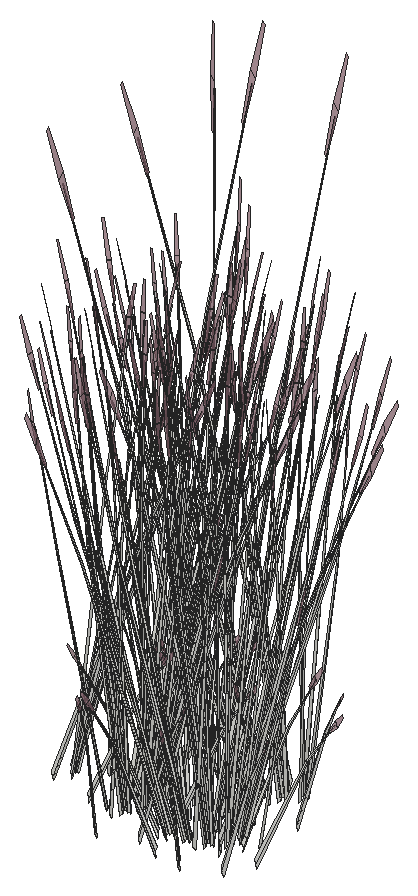
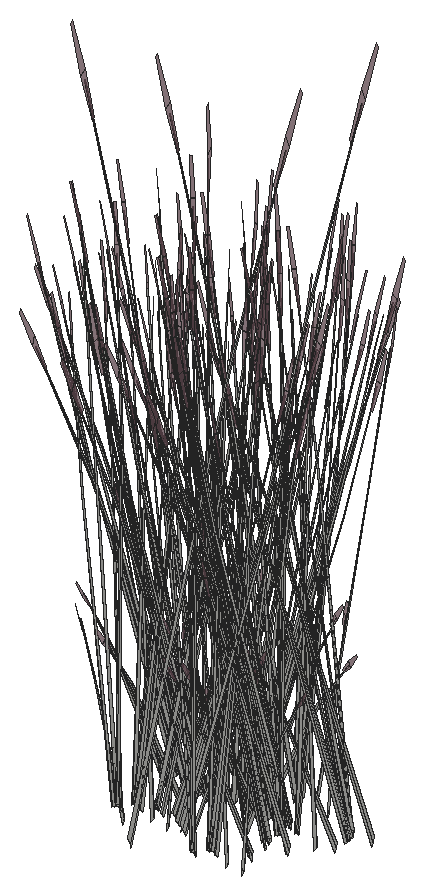
# SketchUp Ruby script. Lengths in inches.
U = 1.inch
M = Sketchup.active_model
def pt(a) = Geom::Point3d.new(a.map { |v| v * U })
def face(e, loops, mat)
  f = e.add_face(loops[0].map { |a| pt(a) })
  loops[1..].each { |l| e.add_face(l.map { |a| pt(a) }).erase! }
  f.material = f.back_material = mat if mat
  f
end
# faces: each face lists its corners as indices into pts; further lists are holes
def faces(e, pts, list, mat = nil) = list.each { |f| face(e, (f[0].is_a?(Array) ? f : [f]).map { |l| l.map { |i| pts[i] } }, mat) }
# xy, xz, yz: faces in a plane at the given z, y or x. An outline is a flat list of corners, or four numbers for a rectangle; further outlines are holes
def ring(l) = l.size == 4 ? [[l[0], l[1]], [l[2], l[1]], [l[2], l[3]], [l[0], l[3]]] : l.each_slice(2).to_a
def flat(e, list, mat, &to3) = list.each { |f| face(e, (f[0].is_a?(Array) ? f : [f]).map { |l| ring(l).map { |u, v| to3.(u, v) } }, mat) }
def xy(e, z, list, mat = nil) = flat(e, list, mat) { |x, y| [x, y, z] }
def xz(e, y, list, mat = nil) = flat(e, list, mat) { |x, z| [x, y, z] }
def yz(e, x, list, mat = nil) = flat(e, list, mat) { |y, z| [x, y, z] }
def lines(e, pts, list) = list.each { |a, b| e.add_line(pt(pts[a]), pt(pts[b])) }
# prism: a flat outline (further loops are holes) pulled along v
def prism(e, loops, v, mat = nil)
  f = face(e, loops, mat); d = Geom::Vector3d.new(v.map { |x| x * U })
  f.pushpull(f.normal.samedirection?(d) ? d.length : -d.length)
end
def box(e, o, s, mat = nil) = prism(e, [[o, [o[0] + s[0], o[1], o[2]], [o[0] + s[0], o[1] + s[1], o[2]], [o[0], o[1] + s[1], o[2]]]], [0, 0, s[2]], mat)
def at(x, y, z, deg = 0) = Geom::Transformation.translation(pt([x, y, z])) * Geom::Transformation.rotation(ORIGIN, Z_AXIS, deg.degrees)
def axes(o, x, y, z) = Geom::Transformation.new([*x, 0, *y, 0, *z, 0, *pt(o).to_a, 1])
def part(name) = M.definitions.add(name)
# library, detail: a bought-in or finely detailed component or shape, given as its bounding box
def library(name, o, s) = part(name).tap { |d| box(d.entities, o, s) }
def detail(e, o, s) = box(e.add_group.entities, o, s)
def put(e, d, t, mat = nil) = e.add_instance(d, t).tap { |i| i.material = mat if mat }
def group(e, t, mat = nil) = e.add_group.tap { |g| g.transformation = t; g.material = mat if mat }.entities
root = M.entities
M.materials.add("LightPink_Translucent").color = [144, 107, 117]
M.materials["LightPink_Translucent"].alpha = 0.75
c1 = part("blade")
p = [[2.15,0.21,22],[0,0.17,0],[0.09,0.45,0],[2.18,0.31,22],[2.29,0.31,22],[0.38,0.45,0],
  [2.48,0.24,33],[2.49,0.24,33],[2.48,0.22,33]]
faces(c1.entities,p,[[0,1,2,3],[4,5,2,3],[6,3,4,7],[8,0,3,6]])
c2 = part("seeds")
p = [[0.3,-0.1,1.38],[-0.01,-0.03,1.59],[-0.01,-0.03,0.03],[0.14,-0.07,-0.07],[0.29,-0.03,3],[0.15,0.01,3.11]]
faces(c2.entities,p,[[0,1,2,3],[1,0,4,5]],"LightPink_Translucent")
c3 = part("blade with seeds")
put(c3.entities,c1,at(0,0,0))
put(c3.entities,c2,axes([2.4,0.25,30.99],[1.5799,-0.05474,1.17369],[-0.12525,1.92788,0.29478],[-0.07173,-0.02425,1.56792]))
put(root,c3,axes([338.69,15.14,51.43],[0.11542,0.12546,1.51428],[-0.53333,0.10562,0.12244],[-0.12054,-0.19696,0.64734]))
put(root,c3,axes([340.11,15.23,52.4],[-0.24099,-0.31773,-0.62776],[0.49607,-0.17707,0.07576],[-0.05635,-0.15352,0.88802]))
put(root,c3,axes([335.52,15.54,52.4],[0.01314,-0.36145,-0.62776],[0.55324,0.02428,0.07576],[0.05838,-0.15313,0.88802]))
put(root,c3,axes([341.12,15.54,52.4],[0.01314,-0.36145,-0.62776],[0.55324,0.02428,0.07576],[0.05838,-0.15313,0.88802]))
put(root,c3,axes([334.5625,14.96,52],[0.15222,-0.30049,-0.31292],[0.44409,0.08764,0.40398],[-0.04072,-0.12098,0.77298]))
put(root,c3,axes([340.16,14.96,52],[0.15222,-0.30049,-0.31292],[0.44409,0.08764,0.40398],[-0.04072,-0.12098,0.77298]))
put(root,c3,axes([334.9,15.36,51.43],[-0.09401,0.13431,1.51428],[-0.3944,-0.27795,0.12244],[0.17792,-0.17323,0.64734]))
put(root,c3,axes([340.5,15.36,51.43],[-0.09401,0.13431,1.51428],[-0.3944,-0.27795,0.12244],[0.17792,-0.17323,0.64734]))
put(root,c3,axes([339.93,15.17,52.14],[-0.49634,-0.09796,-0.45151],[0.17013,-0.33585,-0.34973],[-0.04551,-0.13522,0.86392]))
put(root,c3,axes([334.64,14.33,50.44],[0.06477,0.22786,1.01491],[-0.35932,-0.1262,0.74569],[0.03867,-0.11667,0.22354]))
put(root,c3,axes([340.24,14.33,50.44],[0.06477,0.22786,1.01491],[-0.35932,-0.1262,0.74569],[0.03867,-0.11667,0.22354]))
put(root,c3,axes([335.41,15.42,52.14],[-0.36145,-0.26255,-0.45151],[0.38183,-0.22994,-0.34973],[0.055,-0.1334,0.86392]))
put(root,c3,axes([341.01,15.42,52.14],[-0.36145,-0.26255,-0.45151],[0.38183,-0.22994,-0.34973],[0.055,-0.1334,0.86392]))
put(root,c3,axes([340.36,15.15,52.45],[-0.49409,0.18193,-0.10745],[-0.24281,-0.32289,-0.59638],[-0.06519,-0.13607,0.90619]))
put(root,c3,axes([335.79,15.56,52.45],[-0.55492,-0.01936,-0.10745],[0.01517,-0.36657,-0.59638],[0.03855,-0.14118,0.90619]))
put(root,c3,axes([341.38,15.56,52.45],[-0.55492,-0.01936,-0.10745],[0.01517,-0.36657,-0.59638],[0.03855,-0.14118,0.90619]))
put(root,c3,axes([335.75,15.32,52],[0.34164,-0.20573,-0.31292],[0.3234,0.23491,0.40398],[0.04921,-0.11936,0.77298]))
put(root,c3,axes([341.35,15.32,52],[0.34164,-0.20573,-0.31292],[0.3234,0.23491,0.40398],[0.04921,-0.11936,0.77298]))
put(root,c3,axes([338.39,14.6,50.44],[0.26338,0.136,1.01491],[-0.38358,0.08175,0.74569],[-0.08207,-0.10452,0.22354]))
put(root,c3,axes([339.03,15.32,52.4],[-0.43054,-0.18887,-0.62776],[0.30598,-0.33097,0.07576],[-0.15599,-0.11277,0.88802]))
put(root,c3,axes([338.88,15.07,52],[-0.07798,-0.31474,-0.31292],[0.44579,-0.08311,0.40398],[-0.11974,-0.09019,0.77298]))
put(root,c3,axes([338.83,15.33,52.14],[-0.49824,0.09289,-0.45151],[-0.08716,-0.35177,-0.34973],[-0.13382,-0.10081,0.86392]))
put(root,c3,axes([336.17,16.17,52.4],[0.26374,-0.30832,-0.62776],[0.46217,0.21911,0.07576],[0.15748,-0.11171,0.88802]))
put(root,c3,axes([341.77,16.17,52.4],[0.26374,-0.30832,-0.62776],[0.46217,0.21911,0.07576],[0.15748,-0.11171,0.88802]))
put(root,c3,axes([336.16,16.03,52.14],[-0.12971,-0.3568,-0.45151],[0.49122,-0.06241,-0.34973],[0.14077,-0.09583,0.86392]))
put(root,c3,axes([341.76,16.03,52.14],[-0.12971,-0.3568,-0.45151],[0.49122,-0.06241,-0.34973],[0.14077,-0.09583,0.86392]))
put(root,c3,axes([336.39,16.28,52.45],[-0.46706,-0.21546,-0.10745],[0.26908,-0.31203,-0.59638],[0.13196,-0.10846,0.90619]))
put(root,c3,axes([341.99,16.28,52.45],[-0.46706,-0.21546,-0.10745],[0.26908,-0.31203,-0.59638],[0.13196,-0.10846,0.90619]))
put(root,c3,axes([340.06,17.46,50.9375],[0.43633,0.15757,1.33654],[-0.42745,0.33945,0.52853],[-0.19146,-0.20119,1.12046]))
put(root,c3,axes([336.76,15.32,50.44],[-0.16818,0.19891,1.01491],[-0.14456,-0.26725,0.74569],[0.1389,-0.06697,0.22354]))
put(root,c3,axes([342.36,15.32,50.44],[-0.16818,0.19891,1.01491],[-0.14456,-0.26725,0.74569],[0.1389,-0.06697,0.22354]))
put(root,c3,axes([336.52,16.0625,52],[0.43951,-0.05584,-0.31292],[0.11606,0.31924,0.40398],[0.12595,-0.08575,0.77298]))
put(root,c3,axes([342.12,16.0625,52],[0.43951,-0.05584,-0.31292],[0.11606,0.31924,0.40398],[0.12595,-0.08575,0.77298]))
put(root,c3,axes([337.85,15.625,52],[-0.28729,-0.24465,-0.31292],[0.32804,-0.23159,0.40398],[-0.16667,-0.03524,0.77298]))
put(root,c3,axes([337.98,15.87,52.14],[-0.36663,0.25884,-0.45151],[-0.32109,-0.27343,-0.34973],[-0.18628,-0.03938,0.86392]))
put(root,c3,axes([337.16,16.21,50.44],[0.32236,-0.02796,1.01491],[-0.20448,0.24636,0.74569],[-0.1593,-0.03696,0.22354]))
put(root,c3,axes([332.66,18.94,52.4],[0.01314,-0.36145,-0.62776],[0.55324,0.02428,0.07576],[0.05838,-0.15313,0.88802]))
put(root,c3,axes([338.18,15.6,52.45],[-0.02704,0.39739,-0.10745],[-0.51189,-0.01086,-0.59638],[-0.19715,-0.0276,0.90619]))
put(root,c3,axes([330.75,17.12,52.45],[-0.25405,-0.35383,-0.10745],[0.45089,-0.17388,-0.59638],[0.19001,-0.04668,0.90619]))
put(root,c3,axes([336.41,17.12,52.45],[-0.25405,-0.35383,-0.10745],[0.45089,-0.17388,-0.59638],[0.19001,-0.04668,0.90619]))
put(root,c3,axes([342.01,17.12,52.45],[-0.25405,-0.35383,-0.10745],[0.45089,-0.17388,-0.59638],[0.19001,-0.04668,0.90619]))
put(root,c3,axes([330.73,16.82,52.14],[0.13679,-0.35544,-0.45151],[0.46898,0.12183,-0.34973],[0.18882,-0.03259,0.86392]))
put(root,c3,axes([336.39,16.82,52.14],[0.13679,-0.35544,-0.45151],[0.46898,0.12183,-0.34973],[0.18882,-0.03259,0.86392]))
put(root,c3,axes([341.98,16.82,52.14],[0.13679,-0.35544,-0.45151],[0.46898,0.12183,-0.34973],[0.18882,-0.03259,0.86392]))
put(root,c3,axes([332.04,18.76,51.43],[-0.09401,0.13431,1.51428],[-0.3944,-0.27795,0.12244],[0.17792,-0.17323,0.64734]))
put(root,c3,axes([330.64,16.95,52.4],[0.44368,-0.17257,-0.62776],[0.24726,0.35524,0.07576],[0.21437,-0.04035,0.88802]))
put(root,c3,axes([336.3,16.95,52.4],[0.44368,-0.17257,-0.62776],[0.24726,0.35524,0.07576],[0.21437,-0.04035,0.88802]))
put(root,c3,axes([341.9,16.95,52.4],[0.44368,-0.17257,-0.62776],[0.24726,0.35524,0.07576],[0.21437,-0.04035,0.88802]))
put(root,c3,axes([332.89,18.72,52],[0.34164,-0.20573,-0.31292],[0.3234,0.23491,0.40398],[0.04921,-0.11936,0.77298]))
put(root,c3,axes([331.02,16.98,52],[0.41962,0.10901,-0.31292],[-0.12239,0.31802,0.40398],[0.16894,-0.02916,0.77298]))
put(root,c3,axes([336.68,16.98,52],[0.41962,0.10901,-0.31292],[-0.12239,0.31802,0.40398],[0.16894,-0.02916,0.77298]))
put(root,c3,axes([342.27,16.98,52],[0.41962,0.10901,-0.31292],[-0.12239,0.31802,0.40398],[0.16894,-0.02916,0.77298]))
put(root,c3,axes([329.875,16.59,51.43],[-0.20943,0.00885,1.51428],[0.13893,-0.38357,0.12244],[0.29846,0.02372,0.64734]))
put(root,c3,axes([335.53,16.59,51.43],[-0.20943,0.00885,1.51428],[0.13893,-0.38357,0.12244],[0.29846,0.02372,0.64734]))
put(root,c3,axes([341.13,16.59,51.43],[-0.20943,0.00885,1.51428],[0.13893,-0.38357,0.12244],[0.29846,0.02372,0.64734]))
put(root,c3,axes([333.3125,19.57,52.4],[0.26374,-0.30832,-0.62776],[0.46217,0.21911,0.07576],[0.15748,-0.11171,0.88802]))
put(root,c3,axes([333.3,19.43,52.14],[-0.12971,-0.3568,-0.45151],[0.49122,-0.06241,-0.34973],[0.14077,-0.09583,0.86392]))
put(root,c3,axes([333.53,19.68,52.45],[-0.46706,-0.21546,-0.10745],[0.26908,-0.31203,-0.59638],[0.13196,-0.10846,0.90619]))
put(root,c3,axes([331.91,17.04,50.44],[-0.31197,0.06451,1.01491],[0.14684,-0.26661,0.74569],[0.1655,0.01824,0.22354]))
put(root,c3,axes([337.57,17.04,50.44],[-0.31197,0.06451,1.01491],[0.14684,-0.26661,0.74569],[0.1655,0.01824,0.22354]))
put(root,c3,axes([343.16,17.04,50.44],[-0.31197,0.06451,1.01491],[0.14684,-0.26661,0.74569],[0.1655,0.01824,0.22354]))
put(root,c3,axes([337.63,16.64,52.14],[-0.13679,0.35544,-0.45151],[-0.46898,-0.12183,-0.34973],[-0.18882,0.03259,0.86392]))
put(root,c3,axes([337.61,16.33,52.45],[0.25405,0.35383,-0.10745],[-0.45089,0.17388,-0.59638],[-0.19001,0.04668,0.90619]))
put(root,c3,axes([333.9,18.72,50.44],[-0.16818,0.19891,1.01491],[-0.14456,-0.26725,0.74569],[0.1389,-0.06697,0.22354]))
put(root,c3,axes([337.02,17.87,51.47],[-0.09664,-0.32847,-0.03085],[0.45676,-0.07551,-0.13989],[0.09538,0.02082,0.4614]))
put(root,c3,axes([342.62,17.87,51.47],[-0.09664,-0.32847,-0.03085],[0.45676,-0.07551,-0.13989],[0.09538,0.02082,0.4614]))
put(root,c3,axes([330.18,17.86,52.45],[0.02704,-0.39739,-0.10745],[0.51189,0.01086,-0.59638],[0.19715,0.0276,0.90619]))
put(root,c3,axes([335.84,17.86,52.45],[0.02704,-0.39739,-0.10745],[0.51189,0.01086,-0.59638],[0.19715,0.0276,0.90619]))
put(root,c3,axes([341.4375,17.86,52.45],[0.02704,-0.39739,-0.10745],[0.51189,0.01086,-0.59638],[0.19715,0.0276,0.90619]))
put(root,c3,axes([333.66,19.46,52],[0.43951,-0.05584,-0.31292],[0.11606,0.31924,0.40398],[0.12595,-0.08575,0.77298]))
put(root,c3,axes([338.69,21.41,51.43],[0.11542,0.12546,1.51428],[-0.53333,0.10562,0.12244],[-0.12054,-0.19696,0.64734]))
put(root,c3,axes([340.11,21.5,52.4],[-0.24099,-0.31773,-0.62776],[0.49607,-0.17707,0.07576],[-0.05635,-0.15352,0.88802]))
put(root,c3,axes([330.21,17.67,52.4],[0.50473,0.00941,-0.62776],[-0.0339,0.39618,0.07576],[0.21383,0.04181,0.88802]))
put(root,c3,axes([335.86,17.67,52.4],[0.50473,0.00941,-0.62776],[-0.0339,0.39618,0.07576],[0.21383,0.04181,0.88802]))
put(root,c3,axes([341.46,17.67,52.4],[0.50473,0.00941,-0.62776],[-0.0339,0.39618,0.07576],[0.21383,0.04181,0.88802]))
put(root,c3,axes([341.12,21.8125,52.4],[0.01314,-0.36145,-0.62776],[0.55324,0.02428,0.07576],[0.05838,-0.15313,0.88802]))
put(root,c3,axes([340.16,21.23,52],[0.15222,-0.30049,-0.31292],[0.44409,0.08764,0.40398],[-0.04072,-0.12098,0.77298]))
put(root,c3,axes([340.5,21.63,51.43],[-0.09401,0.13431,1.51428],[-0.3944,-0.27795,0.12244],[0.17792,-0.17323,0.64734]))
put(root,c3,axes([339.93,21.4375,52.14],[-0.49634,-0.09796,-0.45151],[0.17013,-0.33585,-0.34973],[-0.04551,-0.13522,0.86392]))
put(root,c3,axes([340.24,20.6,50.44],[0.06477,0.22786,1.01491],[-0.35932,-0.1262,0.74569],[0.03867,-0.11667,0.22354]))
put(root,c3,axes([341.01,21.69,52.14],[-0.36145,-0.26255,-0.45151],[0.38183,-0.22994,-0.34973],[0.055,-0.1334,0.86392]))
put(root,c3,axes([336.7,18.16,50.44],[0.21042,-0.1771,1.01491],[0.08303,0.28036,0.74569],[-0.15207,0.0502,0.22354]))
put(root,c3,axes([330.51,17.83,52],[0.28729,0.24465,-0.31292],[-0.32804,0.23159,0.40398],[0.16667,0.03524,0.77298]))
put(root,c3,axes([336.17,17.83,52],[0.28729,0.24465,-0.31292],[-0.32804,0.23159,0.40398],[0.16667,0.03524,0.77298]))
put(root,c3,axes([341.77,17.83,52],[0.28729,0.24465,-0.31292],[-0.32804,0.23159,0.40398],[0.16667,0.03524,0.77298]))
put(root,c3,axes([337.49,17.39,52],[-0.43951,0.05584,-0.31292],[-0.11606,-0.31924,0.40398],[-0.12595,0.08575,0.77298]))
put(root,c3,axes([333.55,20.52,52.45],[-0.25405,-0.35383,-0.10745],[0.45089,-0.17388,-0.59638],[0.19001,-0.04668,0.90619]))
put(root,c3,axes([333.53,20.22,52.14],[0.13679,-0.35544,-0.45151],[0.46898,0.12183,-0.34973],[0.18882,-0.03259,0.86392]))
put(root,c3,axes([340.36,21.42,52.45],[-0.49409,0.18193,-0.10745],[-0.24281,-0.32289,-0.59638],[-0.06519,-0.13607,0.90619]))
put(root,c3,axes([341.38,21.83,52.45],[-0.55492,-0.01936,-0.10745],[0.01517,-0.36657,-0.59638],[0.03855,-0.14118,0.90619]))
put(root,c3,axes([341.35,21.6,52],[0.34164,-0.20573,-0.31292],[0.3234,0.23491,0.40398],[0.04921,-0.11936,0.77298]))
put(root,c3,axes([338.39,20.87,50.44],[0.26338,0.136,1.01491],[-0.38358,0.08175,0.74569],[-0.08207,-0.10452,0.22354]))
put(root,c3,axes([339.03,21.59,52.4],[-0.43054,-0.18887,-0.62776],[0.30598,-0.33097,0.07576],[-0.15599,-0.11277,0.88802]))
put(root,c3,axes([338.88,21.34,52],[-0.07798,-0.31474,-0.31292],[0.44579,-0.08311,0.40398],[-0.11974,-0.09019,0.77298]))
put(root,c3,axes([335.14,17.2,51.43],[-0.18755,-0.06732,1.51428],[0.38813,-0.28243,0.12244],[0.24191,0.12741,0.64734]))
put(root,c3,axes([340.73,17.2,51.43],[-0.18755,-0.06732,1.51428],[0.38813,-0.28243,0.12244],[0.24191,0.12741,0.64734]))
put(root,c3,axes([335.17,16.32,51.95],[-0.4363,-0.20303,1.22187],[0.46069,-0.31611,0.5272],[0.14077,0.1905,1.18105]))
put(root,c3,axes([340.77,16.32,51.95],[-0.4363,-0.20303,1.22187],[0.46069,-0.31611,0.5272],[0.14077,0.1905,1.18105]))
put(root,c3,axes([333.4375,20.35,52.4],[0.44368,-0.17257,-0.62776],[0.24726,0.35524,0.07576],[0.21437,-0.04035,0.88802]))
put(root,c3,axes([337.625,17.17,52.45],[0.46706,0.21546,-0.10745],[-0.26908,0.31203,-0.59638],[-0.13196,0.10846,0.90619]))
put(root,c3,axes([335.83,17.97,50.44],[-0.28429,-0.11236,1.01491],[0.36709,-0.11416,0.74569],[0.09901,0.0967,0.22354]))
put(root,c3,axes([341.43,17.97,50.44],[-0.28429,-0.11236,1.01491],[0.36709,-0.11416,0.74569],[0.09901,0.0967,0.22354]))
put(root,c3,axes([334.83,18.29,52.45],[0.30087,-0.33447,-0.10745],[0.43572,0.19269,-0.59638],[0.15146,0.0945,0.90619]))
put(root,c3,axes([340.43,18.29,52.45],[0.30087,-0.33447,-0.10745],[0.43572,0.19269,-0.59638],[0.15146,0.0945,0.90619]))
put(root,c3,axes([338.25,17.08,51.43],[0.12611,-0.12006,1.51428],[0.31843,0.32408,0.12244],[-0.2184,0.14759,0.64734]))
put(root,c3,axes([337.86,17.43,52.14],[0.12971,0.3568,-0.45151],[-0.49122,0.06241,-0.34973],[-0.14077,0.09583,0.86392]))
put(root,c3,axes([338.83,21.6,52.14],[-0.49824,0.09289,-0.45151],[-0.08716,-0.35177,-0.34973],[-0.13382,-0.10081,0.86392]))
put(root,c3,axes([340.74,16.7,50.51],[-0.01379,-0.36791,1.24828],[0.62424,0.09537,0.52853],[-0.14764,0.20132,1.17828]))
put(root,c3,axes([335.12,23.14,52.4],[0.01314,-0.36145,-0.62776],[0.55324,0.02428,0.07576],[0.05838,-0.15313,0.88802]))
put(root,c3,axes([335.1875,18.125,52.14],[0.49824,-0.09289,-0.45151],[0.08716,0.35177,-0.34973],[0.13382,0.10081,0.86392]))
put(root,c3,axes([340.79,18.125,52.14],[0.49824,-0.09289,-0.45151],[0.08716,0.35177,-0.34973],[0.13382,0.10081,0.86392]))
put(root,c3,axes([334.5,22.96,51.43],[-0.09401,0.13431,1.51428],[-0.3944,-0.27795,0.12244],[0.17792,-0.17323,0.64734]))
put(root,c3,axes([341.77,22.44,52.4],[0.26374,-0.30832,-0.62776],[0.46217,0.21911,0.07576],[0.15748,-0.11171,0.88802]))
put(root,c3,axes([341.76,22.3,52.14],[-0.12971,-0.3568,-0.45151],[0.49122,-0.06241,-0.34973],[0.14077,-0.09583,0.86392]))
put(root,c3,axes([333.82,20.38,52],[0.41962,0.10901,-0.31292],[-0.12239,0.31802,0.40398],[0.16894,-0.02916,0.77298]))
put(root,c3,axes([334.24,21.92,50.44],[0.06477,0.22786,1.01491],[-0.35932,-0.1262,0.74569],[0.03867,-0.11667,0.22354]))
put(root,c3,axes([335.01,23.02,52.14],[-0.36145,-0.26255,-0.45151],[0.38183,-0.22994,-0.34973],[0.055,-0.1334,0.86392]))
put(root,c3,axes([341.99,22.55,52.45],[-0.46706,-0.21546,-0.10745],[0.26908,-0.31203,-0.59638],[0.13196,-0.10846,0.90619]))
put(root,c3,axes([332.67,19.99,51.43],[-0.20943,0.00885,1.51428],[0.13893,-0.38357,0.12244],[0.29846,0.02372,0.64734]))
put(root,c3,axes([338.16,17.37,51.43],[0.09401,-0.13431,1.51428],[0.3944,0.27795,0.12244],[-0.17792,0.17323,0.64734]))
put(root,c3,axes([340.06,23.73,50.9375],[0.43633,0.15757,1.33654],[-0.42745,0.33945,0.52853],[-0.19146,-0.20119,1.12046]))
put(root,c3,axes([335.38,23.16,52.45],[-0.55492,-0.01936,-0.10745],[0.01517,-0.36657,-0.59638],[0.03855,-0.14118,0.90619]))
put(root,c3,axes([335.35,22.92,52],[0.34164,-0.20573,-0.31292],[0.3234,0.23491,0.40398],[0.04921,-0.11936,0.77298]))
put(root,c3,axes([338.27,18.13,52],[-0.34164,0.20573,-0.31292],[-0.3234,-0.23491,0.40398],[-0.04921,0.11936,0.77298]))
put(root,c3,axes([333.66,18.3,52.45],[0.49409,-0.18193,-0.10745],[0.24281,0.32289,-0.59638],[0.06519,0.13607,0.90619]))
put(root,c3,axes([339.25,18.3,52.45],[0.49409,-0.18193,-0.10745],[0.24281,0.32289,-0.59638],[0.06519,0.13607,0.90619]))
put(root,c3,axes([342.36,21.59,50.44],[-0.16818,0.19891,1.01491],[-0.14456,-0.26725,0.74569],[0.1389,-0.06697,0.22354]))
put(root,c3,axes([338.48,18.93,50.44],[-0.01307,-0.23234,1.01491],[0.32652,0.16572,0.74569],[-0.06422,0.11074,0.22354]))
put(root,c3,axes([342.12,22.33,52],[0.43951,-0.05584,-0.31292],[0.11606,0.31924,0.40398],[0.12595,-0.08575,0.77298]))
put(root,c3,axes([334.71,20.45,50.44],[-0.31197,0.06451,1.01491],[0.14684,-0.26661,0.74569],[0.1655,0.01824,0.22354]))
put(root,c3,axes([337.85,21.9,52],[-0.28729,-0.24465,-0.31292],[0.32804,-0.23159,0.40398],[-0.16667,-0.03524,0.77298]))
put(root,c3,axes([338.61,18.03,52.42],[0.36145,0.26255,-0.50118],[-0.38183,0.22994,-0.3882],[-0.055,0.1334,0.95895]))
put(root,c3,axes([334.08,18.29,52.14],[0.49634,0.09796,-0.45151],[-0.17013,0.33585,-0.34973],[0.04551,0.13522,0.86392]))
put(root,c3,axes([339.68,18.29,52.14],[0.49634,0.09796,-0.45151],[-0.17013,0.33585,-0.34973],[0.04551,0.13522,0.86392]))
put(root,c3,axes([334.36,17.59,51.43],[-0.11542,-0.12546,1.51428],[0.53333,-0.10562,0.12244],[0.12054,0.19696,0.64734]))
put(root,c3,axes([339.96,17.59,51.43],[-0.11542,-0.12546,1.51428],[0.53333,-0.10562,0.12244],[0.12054,0.19696,0.64734]))
put(root,c3,axes([333.86,18.49,52],[-0.15222,0.30049,-0.31292],[-0.44409,-0.08764,0.40398],[0.04072,0.12098,0.77298]))
put(root,c3,axes([339.45,18.49,52],[-0.15222,0.30049,-0.31292],[-0.44409,-0.08764,0.40398],[0.04072,0.12098,0.77298]))
put(root,c3,axes([334.16,21.27,51.47],[-0.09664,-0.32847,-0.03085],[0.45676,-0.07551,-0.13989],[0.09538,0.02082,0.4614]))
put(root,c3,axes([332.98,21.26,52.45],[0.02704,-0.39739,-0.10745],[0.51189,0.01086,-0.59638],[0.19715,0.0276,0.90619]))
put(root,c3,axes([338.49,17.91,52.72],[-0.01314,0.36145,-0.69681],[-0.55324,-0.02428,0.08409],[-0.05838,0.15313,0.9857]))
put(root,c3,axes([339.02,17.66,51.43],[-0.01236,-0.14998,1.51428],[0.53562,0.09949,0.12244],[-0.03313,0.21373,0.64734]))
put(root,c3,axes([335.77,23.77,52.4],[0.26374,-0.30832,-0.62776],[0.46217,0.21911,0.07576],[0.15748,-0.11171,0.88802]))
put(root,c3,axes([335.76,23.625,52.14],[-0.12971,-0.3568,-0.45151],[0.49122,-0.06241,-0.34973],[0.14077,-0.09583,0.86392]))
put(root,c3,axes([333.9,18.22,52.4],[0.24099,0.31773,-0.62776],[-0.49607,0.17707,0.07576],[0.05635,0.15352,0.88802]))
put(root,c3,axes([339.5,18.22,52.4],[0.24099,0.31773,-0.62776],[-0.49607,0.17707,0.07576],[0.05635,0.15352,0.88802]))
put(root,c3,axes([335.99,23.88,52.45],[-0.46706,-0.21546,-0.10745],[0.26908,-0.31203,-0.59638],[0.13196,-0.10846,0.90619]))
put(root,c3,axes([337.98,22.14,52.14],[-0.36663,0.25884,-0.45151],[-0.32109,-0.27343,-0.34973],[-0.18628,-0.03938,0.86392]))
